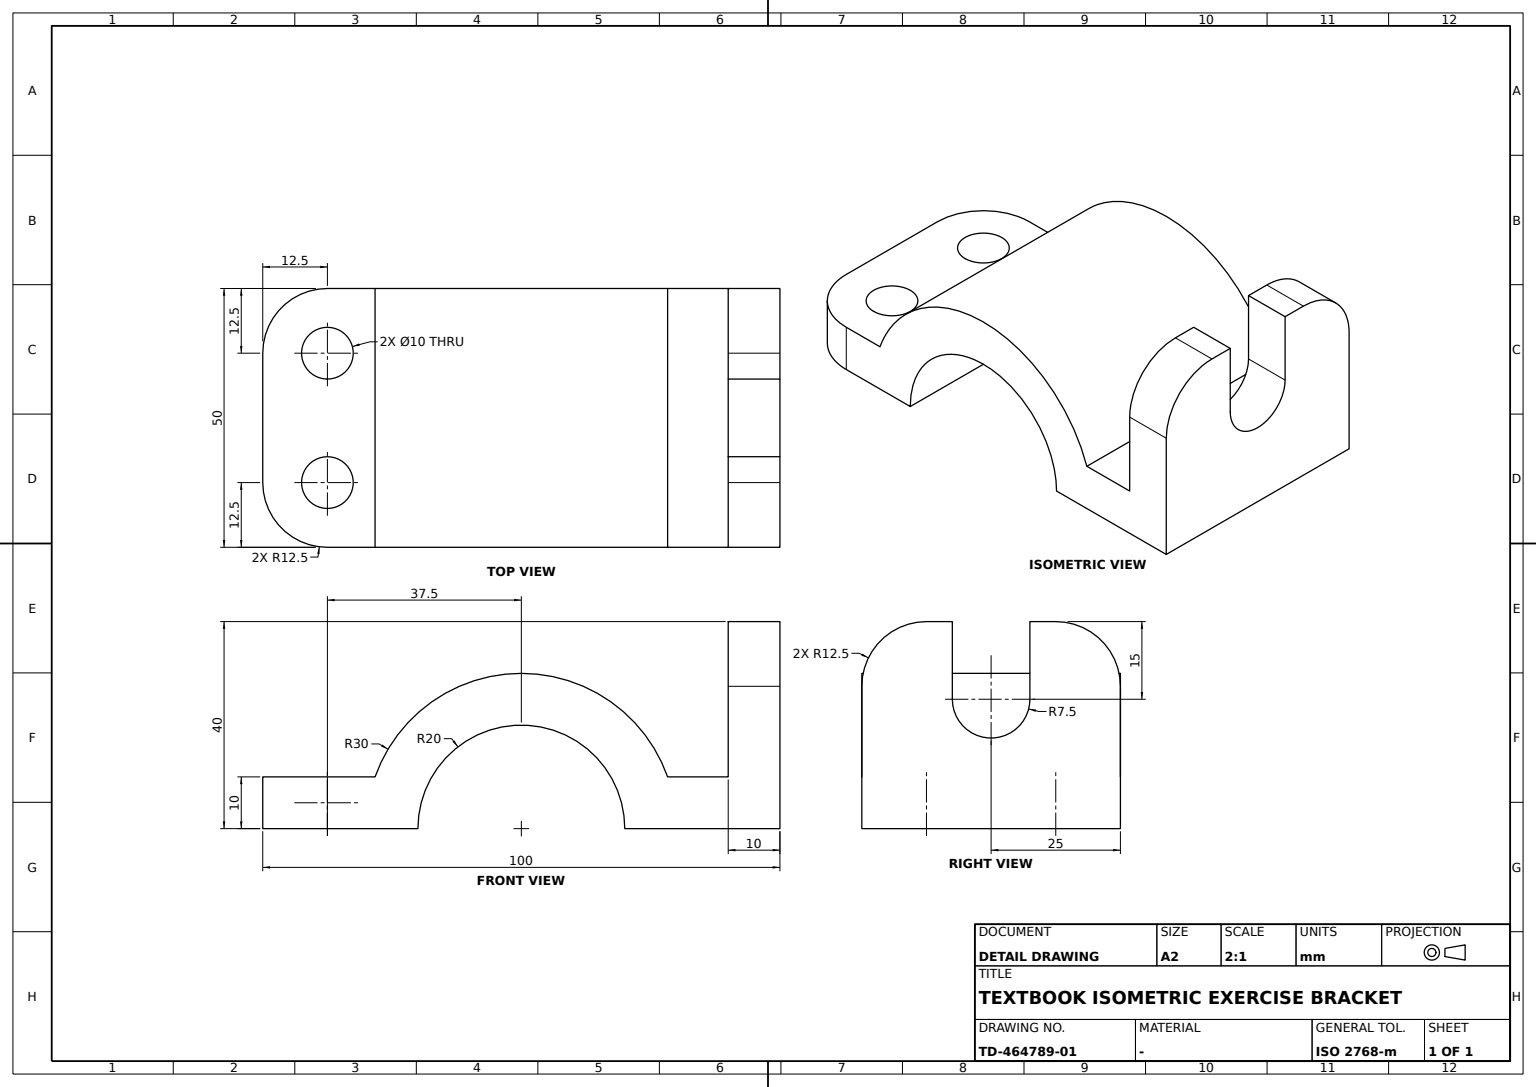
ISO-10303-21;
HEADER;
FILE_DESCRIPTION((''),'2;1');
FILE_NAME('','',(''),(''),'','','');
FILE_SCHEMA(('AUTOMOTIVE_DESIGN'));
ENDSEC;
DATA;
#1=APPLICATION_CONTEXT('');
#2=PRODUCT_CONTEXT('',#1,'mechanical');
#3=PRODUCT('','','',(#2));
#4=PRODUCT_DEFINITION_FORMATION('','',#3);
#5=PRODUCT_DEFINITION_CONTEXT('',#1,'design');
#6=PRODUCT_DEFINITION('','',#4,#5);
#7=PRODUCT_DEFINITION_SHAPE('','',#6);
#8=(LENGTH_UNIT()NAMED_UNIT(*)SI_UNIT(.MILLI.,.METRE.));
#9=(NAMED_UNIT(*)PLANE_ANGLE_UNIT()SI_UNIT($,.RADIAN.));
#10=(NAMED_UNIT(*)SI_UNIT($,.STERADIAN.)SOLID_ANGLE_UNIT());
#11=UNCERTAINTY_MEASURE_WITH_UNIT(LENGTH_MEASURE(1.E-05),#8,'distance_accuracy_value','');
#12=(GEOMETRIC_REPRESENTATION_CONTEXT(3)GLOBAL_UNCERTAINTY_ASSIGNED_CONTEXT((#11))GLOBAL_UNIT_ASSIGNED_CONTEXT((#8,#9,#10))REPRESENTATION_CONTEXT('',''));
#13=CARTESIAN_POINT('',(12.5,40.,40.));
#14=VERTEX_POINT('',#13);
#15=CARTESIAN_POINT('',(25.,40.,27.5));
#16=VERTEX_POINT('',#15);
#17=CARTESIAN_POINT('',(12.5,40.,27.5));
#18=DIRECTION('',(0.,1.,0.));
#19=DIRECTION('',(0.,0.,-1.));
#20=AXIS2_PLACEMENT_3D('',#17,#18,#19);
#21=CIRCLE('',#20,12.5);
#22=EDGE_CURVE('',#14,#16,#21,.T.);
#23=ORIENTED_EDGE('',*,*,#22,.F.);
#24=CARTESIAN_POINT('',(7.5,40.,40.));
#25=VERTEX_POINT('',#24);
#26=CARTESIAN_POINT('',(10.,40.,40.));
#27=DIRECTION('',(1.,0.,0.));
#28=VECTOR('',#27,1000.);
#29=LINE('',#26,#28);
#30=EDGE_CURVE('',#25,#14,#29,.T.);
#31=ORIENTED_EDGE('',*,*,#30,.F.);
#32=CARTESIAN_POINT('',(7.5,40.,25.));
#33=VERTEX_POINT('',#32);
#34=CARTESIAN_POINT('',(7.5,40.,32.5));
#35=VECTOR('',#19,1000.);
#36=LINE('',#34,#35);
#37=EDGE_CURVE('',#25,#33,#36,.T.);
#38=ORIENTED_EDGE('',*,*,#37,.T.);
#39=CARTESIAN_POINT('',(-7.5,40.,25.));
#40=VERTEX_POINT('',#39);
#41=CARTESIAN_POINT('',(0.,40.,25.));
#42=DIRECTION('',(0.,-1.,0.));
#43=AXIS2_PLACEMENT_3D('',#41,#42,#19);
#44=CIRCLE('',#43,7.5);
#45=EDGE_CURVE('',#40,#33,#44,.T.);
#46=ORIENTED_EDGE('',*,*,#45,.F.);
#47=CARTESIAN_POINT('',(-7.5,40.,40.));
#48=VERTEX_POINT('',#47);
#49=CARTESIAN_POINT('',(-7.5,40.,32.5));
#50=LINE('',#49,#35);
#51=EDGE_CURVE('',#48,#40,#50,.T.);
#52=ORIENTED_EDGE('',*,*,#51,.F.);
#53=CARTESIAN_POINT('',(-12.5,40.,40.));
#54=VERTEX_POINT('',#53);
#55=CARTESIAN_POINT('',(-10.,40.,40.));
#56=LINE('',#55,#28);
#57=EDGE_CURVE('',#54,#48,#56,.T.);
#58=ORIENTED_EDGE('',*,*,#57,.F.);
#59=CARTESIAN_POINT('',(-25.,40.,27.5));
#60=VERTEX_POINT('',#59);
#61=CARTESIAN_POINT('',(-12.5,40.,27.5));
#62=AXIS2_PLACEMENT_3D('',#61,#18,#19);
#63=CIRCLE('',#62,12.5);
#64=EDGE_CURVE('',#60,#54,#63,.T.);
#65=ORIENTED_EDGE('',*,*,#64,.F.);
#66=CARTESIAN_POINT('',(-25.,40.,10.));
#67=VERTEX_POINT('',#66);
#68=CARTESIAN_POINT('',(-25.,40.,18.75));
#69=LINE('',#68,#35);
#70=EDGE_CURVE('',#60,#67,#69,.T.);
#71=ORIENTED_EDGE('',*,*,#70,.T.);
#72=CARTESIAN_POINT('',(25.,40.,10.));
#73=VERTEX_POINT('',#72);
#74=CARTESIAN_POINT('',(0.,40.,10.));
#75=LINE('',#74,#28);
#76=EDGE_CURVE('',#67,#73,#75,.T.);
#77=ORIENTED_EDGE('',*,*,#76,.T.);
#78=CARTESIAN_POINT('',(25.,40.,18.75));
#79=LINE('',#78,#35);
#80=EDGE_CURVE('',#16,#73,#79,.T.);
#81=ORIENTED_EDGE('',*,*,#80,.F.);
#82=EDGE_LOOP('',(#23,#31,#38,#46,#52,#58,#65,#71,#77,#81));
#83=FACE_OUTER_BOUND('',#82,.T.);
#84=CARTESIAN_POINT('',(0.,40.,40.));
#85=AXIS2_PLACEMENT_3D('',#84,#42,#19);
#86=PLANE('',#85);
#87=ADVANCED_FACE('',(#83),#86,.T.);
#88=CARTESIAN_POINT('',(-25.,-37.5,0.));
#89=VERTEX_POINT('',#88);
#90=CARTESIAN_POINT('',(-12.5,-50.,0.));
#91=VERTEX_POINT('',#90);
#92=CARTESIAN_POINT('',(-12.5,-37.5,0.));
#93=DIRECTION('',(0.,0.,1.));
#94=AXIS2_PLACEMENT_3D('',#92,#93,#18);
#95=CIRCLE('',#94,12.5);
#96=EDGE_CURVE('',#89,#91,#95,.T.);
#97=ORIENTED_EDGE('',*,*,#96,.T.);
#98=CARTESIAN_POINT('',(-12.5,-50.,10.));
#99=VERTEX_POINT('',#98);
#100=CARTESIAN_POINT('',(-12.5,-50.,5.));
#101=LINE('',#100,#35);
#102=EDGE_CURVE('',#99,#91,#101,.T.);
#103=ORIENTED_EDGE('',*,*,#102,.F.);
#104=CARTESIAN_POINT('',(-25.,-37.5,10.));
#105=VERTEX_POINT('',#104);
#106=CARTESIAN_POINT('',(-12.5,-37.5,10.));
#107=AXIS2_PLACEMENT_3D('',#106,#19,#42);
#108=CIRCLE('',#107,12.5);
#109=EDGE_CURVE('',#99,#105,#108,.T.);
#110=ORIENTED_EDGE('',*,*,#109,.T.);
#111=CARTESIAN_POINT('',(-25.,-37.5,5.));
#112=LINE('',#111,#35);
#113=EDGE_CURVE('',#105,#89,#112,.T.);
#114=ORIENTED_EDGE('',*,*,#113,.T.);
#115=EDGE_LOOP('',(#97,#103,#110,#114));
#116=FACE_OUTER_BOUND('',#115,.T.);
#117=CARTESIAN_POINT('',(-12.5,-37.5,15.));
#118=DIRECTION('',(-1.,0.,0.));
#119=AXIS2_PLACEMENT_3D('',#117,#19,#118);
#120=CYLINDRICAL_SURFACE('',#119,12.5);
#121=ADVANCED_FACE('',(#116),#120,.T.);
#122=CARTESIAN_POINT('',(17.5,-37.5,0.));
#123=VERTEX_POINT('',#122);
#124=CARTESIAN_POINT('',(7.5,-37.5,0.));
#125=VERTEX_POINT('',#124);
#126=CARTESIAN_POINT('',(12.5,-37.5,0.));
#127=AXIS2_PLACEMENT_3D('',#126,#19,#18);
#128=CIRCLE('',#127,5.);
#129=EDGE_CURVE('',#123,#125,#128,.T.);
#130=ORIENTED_EDGE('',*,*,#129,.T.);
#131=CARTESIAN_POINT('',(7.5,-37.5,10.));
#132=VERTEX_POINT('',#131);
#133=CARTESIAN_POINT('',(7.5,-37.5,-2.5));
#134=LINE('',#133,#35);
#135=EDGE_CURVE('',#132,#125,#134,.T.);
#136=ORIENTED_EDGE('',*,*,#135,.F.);
#137=CARTESIAN_POINT('',(17.5,-37.5,10.));
#138=VERTEX_POINT('',#137);
#139=CARTESIAN_POINT('',(12.5,-37.5,10.));
#140=AXIS2_PLACEMENT_3D('',#139,#93,#27);
#141=CIRCLE('',#140,5.);
#142=EDGE_CURVE('',#132,#138,#141,.T.);
#143=ORIENTED_EDGE('',*,*,#142,.T.);
#144=CARTESIAN_POINT('',(17.5,-37.5,-2.5));
#145=LINE('',#144,#35);
#146=EDGE_CURVE('',#138,#123,#145,.T.);
#147=ORIENTED_EDGE('',*,*,#146,.T.);
#148=EDGE_LOOP('',(#130,#136,#143,#147));
#149=FACE_OUTER_BOUND('',#148,.T.);
#150=CARTESIAN_POINT('',(12.5,-37.5,-2.5));
#151=AXIS2_PLACEMENT_3D('',#150,#19,#27);
#152=CYLINDRICAL_SURFACE('',#151,5.);
#153=ADVANCED_FACE('',(#149),#152,.F.);
#154=CARTESIAN_POINT('',(12.5,50.,40.));
#155=VERTEX_POINT('',#154);
#156=CARTESIAN_POINT('',(12.5,45.,40.));
#157=VECTOR('',#42,1000.);
#158=LINE('',#156,#157);
#159=EDGE_CURVE('',#155,#14,#158,.T.);
#160=ORIENTED_EDGE('',*,*,#159,.T.);
#161=ORIENTED_EDGE('',*,*,#22,.T.);
#162=CARTESIAN_POINT('',(25.,50.,27.5));
#163=VERTEX_POINT('',#162);
#164=CARTESIAN_POINT('',(25.,45.,27.5));
#165=LINE('',#164,#157);
#166=EDGE_CURVE('',#163,#16,#165,.T.);
#167=ORIENTED_EDGE('',*,*,#166,.F.);
#168=CARTESIAN_POINT('',(12.5,50.,27.5));
#169=AXIS2_PLACEMENT_3D('',#168,#42,#93);
#170=CIRCLE('',#169,12.5);
#171=EDGE_CURVE('',#163,#155,#170,.T.);
#172=ORIENTED_EDGE('',*,*,#171,.T.);
#173=EDGE_LOOP('',(#160,#161,#167,#172));
#174=FACE_OUTER_BOUND('',#173,.T.);
#175=CARTESIAN_POINT('',(12.5,0.,27.5));
#176=AXIS2_PLACEMENT_3D('',#175,#18,#93);
#177=CYLINDRICAL_SURFACE('',#176,12.5);
#178=ADVANCED_FACE('',(#174),#177,.T.);
#179=CARTESIAN_POINT('',(12.5,-50.,0.));
#180=VERTEX_POINT('',#179);
#181=CARTESIAN_POINT('',(25.,-37.5,0.));
#182=VERTEX_POINT('',#181);
#183=AXIS2_PLACEMENT_3D('',#126,#93,#18);
#184=CIRCLE('',#183,12.5);
#185=EDGE_CURVE('',#180,#182,#184,.T.);
#186=ORIENTED_EDGE('',*,*,#185,.T.);
#187=CARTESIAN_POINT('',(25.,-37.5,10.));
#188=VERTEX_POINT('',#187);
#189=CARTESIAN_POINT('',(25.,-37.5,5.));
#190=LINE('',#189,#35);
#191=EDGE_CURVE('',#188,#182,#190,.T.);
#192=ORIENTED_EDGE('',*,*,#191,.F.);
#193=CARTESIAN_POINT('',(12.5,-50.,10.));
#194=VERTEX_POINT('',#193);
#195=AXIS2_PLACEMENT_3D('',#139,#19,#42);
#196=CIRCLE('',#195,12.5);
#197=EDGE_CURVE('',#188,#194,#196,.T.);
#198=ORIENTED_EDGE('',*,*,#197,.T.);
#199=CARTESIAN_POINT('',(12.5,-50.,5.));
#200=LINE('',#199,#35);
#201=EDGE_CURVE('',#194,#180,#200,.T.);
#202=ORIENTED_EDGE('',*,*,#201,.T.);
#203=EDGE_LOOP('',(#186,#192,#198,#202));
#204=FACE_OUTER_BOUND('',#203,.T.);
#205=CARTESIAN_POINT('',(12.5,-37.5,15.));
#206=AXIS2_PLACEMENT_3D('',#205,#19,#42);
#207=CYLINDRICAL_SURFACE('',#206,12.5);
#208=ADVANCED_FACE('',(#204),#207,.T.);
#209=CARTESIAN_POINT('',(0.,-50.,0.));
#210=LINE('',#209,#28);
#211=EDGE_CURVE('',#91,#180,#210,.T.);
#212=ORIENTED_EDGE('',*,*,#211,.T.);
#213=ORIENTED_EDGE('',*,*,#201,.F.);
#214=CARTESIAN_POINT('',(0.,-50.,10.));
#215=LINE('',#214,#28);
#216=EDGE_CURVE('',#99,#194,#215,.T.);
#217=ORIENTED_EDGE('',*,*,#216,.F.);
#218=ORIENTED_EDGE('',*,*,#102,.T.);
#219=EDGE_LOOP('',(#212,#213,#217,#218));
#220=FACE_OUTER_BOUND('',#219,.T.);
#221=AXIS2_PLACEMENT_3D('',#209,#18,#93);
#222=PLANE('',#221);
#223=ADVANCED_FACE('',(#220),#222,.F.);
#224=CARTESIAN_POINT('',(7.5,50.,40.));
#225=VERTEX_POINT('',#224);
#226=CARTESIAN_POINT('',(7.5,50.,25.));
#227=VERTEX_POINT('',#226);
#228=CARTESIAN_POINT('',(7.5,50.,32.5));
#229=LINE('',#228,#35);
#230=EDGE_CURVE('',#225,#227,#229,.T.);
#231=ORIENTED_EDGE('',*,*,#230,.F.);
#232=CARTESIAN_POINT('',(10.,50.,40.));
#233=LINE('',#232,#28);
#234=EDGE_CURVE('',#225,#155,#233,.T.);
#235=ORIENTED_EDGE('',*,*,#234,.T.);
#236=ORIENTED_EDGE('',*,*,#171,.F.);
#237=CARTESIAN_POINT('',(25.,50.,0.));
#238=VERTEX_POINT('',#237);
#239=CARTESIAN_POINT('',(25.,50.,13.75));
#240=VECTOR('',#93,1000.);
#241=LINE('',#239,#240);
#242=EDGE_CURVE('',#238,#163,#241,.T.);
#243=ORIENTED_EDGE('',*,*,#242,.F.);
#244=CARTESIAN_POINT('',(-25.,50.,0.));
#245=VERTEX_POINT('',#244);
#246=CARTESIAN_POINT('',(0.,50.,0.));
#247=LINE('',#246,#28);
#248=EDGE_CURVE('',#245,#238,#247,.T.);
#249=ORIENTED_EDGE('',*,*,#248,.F.);
#250=CARTESIAN_POINT('',(-25.,50.,27.5));
#251=VERTEX_POINT('',#250);
#252=CARTESIAN_POINT('',(-25.,50.,13.75));
#253=LINE('',#252,#240);
#254=EDGE_CURVE('',#245,#251,#253,.T.);
#255=ORIENTED_EDGE('',*,*,#254,.T.);
#256=CARTESIAN_POINT('',(-12.5,50.,40.));
#257=VERTEX_POINT('',#256);
#258=CARTESIAN_POINT('',(-12.5,50.,27.5));
#259=AXIS2_PLACEMENT_3D('',#258,#42,#93);
#260=CIRCLE('',#259,12.5);
#261=EDGE_CURVE('',#257,#251,#260,.T.);
#262=ORIENTED_EDGE('',*,*,#261,.F.);
#263=CARTESIAN_POINT('',(-7.5,50.,40.));
#264=VERTEX_POINT('',#263);
#265=CARTESIAN_POINT('',(-10.,50.,40.));
#266=LINE('',#265,#28);
#267=EDGE_CURVE('',#257,#264,#266,.T.);
#268=ORIENTED_EDGE('',*,*,#267,.T.);
#269=CARTESIAN_POINT('',(-7.5,50.,25.));
#270=VERTEX_POINT('',#269);
#271=CARTESIAN_POINT('',(-7.5,50.,32.5));
#272=LINE('',#271,#240);
#273=EDGE_CURVE('',#270,#264,#272,.T.);
#274=ORIENTED_EDGE('',*,*,#273,.F.);
#275=CARTESIAN_POINT('',(0.,50.,25.));
#276=AXIS2_PLACEMENT_3D('',#275,#18,#118);
#277=CIRCLE('',#276,7.5);
#278=EDGE_CURVE('',#227,#270,#277,.T.);
#279=ORIENTED_EDGE('',*,*,#278,.F.);
#280=EDGE_LOOP('',(#231,#235,#236,#243,#249,#255,#262,#268,#274,#279));
#281=FACE_OUTER_BOUND('',#280,.T.);
#282=AXIS2_PLACEMENT_3D('',#246,#18,#93);
#283=PLANE('',#282);
#284=ADVANCED_FACE('',(#281),#283,.T.);
#285=CARTESIAN_POINT('',(25.,-20.,0.));
#286=VERTEX_POINT('',#285);
#287=CARTESIAN_POINT('',(25.,-28.75,0.));
#288=VECTOR('',#18,1000.);
#289=LINE('',#287,#288);
#290=EDGE_CURVE('',#182,#286,#289,.T.);
#291=ORIENTED_EDGE('',*,*,#290,.T.);
#292=CARTESIAN_POINT('',(25.,20.,0.));
#293=VERTEX_POINT('',#292);
#294=CARTESIAN_POINT('',(25.,0.,0.));
#295=AXIS2_PLACEMENT_3D('',#294,#118,#18);
#296=CIRCLE('',#295,20.);
#297=EDGE_CURVE('',#286,#293,#296,.T.);
#298=ORIENTED_EDGE('',*,*,#297,.T.);
#299=CARTESIAN_POINT('',(25.,35.,0.));
#300=LINE('',#299,#288);
#301=EDGE_CURVE('',#293,#238,#300,.T.);
#302=ORIENTED_EDGE('',*,*,#301,.T.);
#303=ORIENTED_EDGE('',*,*,#242,.T.);
#304=ORIENTED_EDGE('',*,*,#166,.T.);
#305=ORIENTED_EDGE('',*,*,#80,.T.);
#306=CARTESIAN_POINT('',(25.,28.284271,10.));
#307=VERTEX_POINT('',#306);
#308=CARTESIAN_POINT('',(25.,34.142136,10.));
#309=LINE('',#308,#157);
#310=EDGE_CURVE('',#73,#307,#309,.T.);
#311=ORIENTED_EDGE('',*,*,#310,.T.);
#312=CARTESIAN_POINT('',(25.,-28.284271,10.));
#313=VERTEX_POINT('',#312);
#314=AXIS2_PLACEMENT_3D('',#294,#27,#18);
#315=CIRCLE('',#314,30.);
#316=EDGE_CURVE('',#307,#313,#315,.T.);
#317=ORIENTED_EDGE('',*,*,#316,.T.);
#318=CARTESIAN_POINT('',(25.,-32.892136,10.));
#319=LINE('',#318,#157);
#320=EDGE_CURVE('',#313,#188,#319,.T.);
#321=ORIENTED_EDGE('',*,*,#320,.T.);
#322=ORIENTED_EDGE('',*,*,#191,.T.);
#323=EDGE_LOOP('',(#291,#298,#302,#303,#304,#305,#311,#317,#321,#322));
#324=FACE_OUTER_BOUND('',#323,.T.);
#325=PLANE('',#314);
#326=ADVANCED_FACE('',(#324),#325,.T.);
#327=ORIENTED_EDGE('',*,*,#278,.T.);
#328=CARTESIAN_POINT('',(-7.5,-0.66,25.));
#329=LINE('',#328,#157);
#330=EDGE_CURVE('',#270,#40,#329,.T.);
#331=ORIENTED_EDGE('',*,*,#330,.T.);
#332=ORIENTED_EDGE('',*,*,#45,.T.);
#333=CARTESIAN_POINT('',(7.5,45.,25.));
#334=LINE('',#333,#157);
#335=EDGE_CURVE('',#227,#33,#334,.T.);
#336=ORIENTED_EDGE('',*,*,#335,.F.);
#337=EDGE_LOOP('',(#327,#331,#332,#336));
#338=FACE_OUTER_BOUND('',#337,.T.);
#339=CARTESIAN_POINT('',(0.,-0.66,25.));
#340=AXIS2_PLACEMENT_3D('',#339,#42,#118);
#341=CYLINDRICAL_SURFACE('',#340,7.5);
#342=ADVANCED_FACE('',(#338),#341,.F.);
#343=EDGE_CURVE('',#138,#132,#141,.T.);
#344=ORIENTED_EDGE('',*,*,#343,.T.);
#345=ORIENTED_EDGE('',*,*,#135,.T.);
#346=EDGE_CURVE('',#125,#123,#128,.T.);
#347=ORIENTED_EDGE('',*,*,#346,.T.);
#348=ORIENTED_EDGE('',*,*,#146,.F.);
#349=EDGE_LOOP('',(#344,#345,#347,#348));
#350=FACE_OUTER_BOUND('',#349,.T.);
#351=ADVANCED_FACE('',(#350),#152,.F.);
#352=CARTESIAN_POINT('',(-12.5,45.,40.));
#353=LINE('',#352,#157);
#354=EDGE_CURVE('',#257,#54,#353,.T.);
#355=ORIENTED_EDGE('',*,*,#354,.T.);
#356=ORIENTED_EDGE('',*,*,#57,.T.);
#357=CARTESIAN_POINT('',(-7.5,45.,40.));
#358=LINE('',#357,#157);
#359=EDGE_CURVE('',#264,#48,#358,.T.);
#360=ORIENTED_EDGE('',*,*,#359,.F.);
#361=ORIENTED_EDGE('',*,*,#267,.F.);
#362=EDGE_LOOP('',(#355,#356,#360,#361));
#363=FACE_OUTER_BOUND('',#362,.T.);
#364=CARTESIAN_POINT('',(0.,50.,40.));
#365=AXIS2_PLACEMENT_3D('',#364,#93,#42);
#366=PLANE('',#365);
#367=ADVANCED_FACE('',(#363),#366,.T.);
#368=ORIENTED_EDGE('',*,*,#310,.F.);
#369=ORIENTED_EDGE('',*,*,#76,.F.);
#370=CARTESIAN_POINT('',(-25.,28.284271,10.));
#371=VERTEX_POINT('',#370);
#372=CARTESIAN_POINT('',(-25.,34.142136,10.));
#373=LINE('',#372,#157);
#374=EDGE_CURVE('',#67,#371,#373,.T.);
#375=ORIENTED_EDGE('',*,*,#374,.T.);
#376=CARTESIAN_POINT('',(0.,28.284271,10.));
#377=LINE('',#376,#28);
#378=EDGE_CURVE('',#371,#307,#377,.T.);
#379=ORIENTED_EDGE('',*,*,#378,.T.);
#380=EDGE_LOOP('',(#368,#369,#375,#379));
#381=FACE_OUTER_BOUND('',#380,.T.);
#382=AXIS2_PLACEMENT_3D('',#74,#93,#42);
#383=PLANE('',#382);
#384=ADVANCED_FACE('',(#381),#383,.T.);
#385=ORIENTED_EDGE('',*,*,#37,.F.);
#386=CARTESIAN_POINT('',(7.5,45.,40.));
#387=LINE('',#386,#157);
#388=EDGE_CURVE('',#225,#25,#387,.T.);
#389=ORIENTED_EDGE('',*,*,#388,.F.);
#390=ORIENTED_EDGE('',*,*,#230,.T.);
#391=ORIENTED_EDGE('',*,*,#335,.T.);
#392=EDGE_LOOP('',(#385,#389,#390,#391));
#393=FACE_OUTER_BOUND('',#392,.T.);
#394=AXIS2_PLACEMENT_3D('',#224,#118,#19);
#395=PLANE('',#394);
#396=ADVANCED_FACE('',(#393),#395,.T.);
#397=ORIENTED_EDGE('',*,*,#330,.F.);
#398=ORIENTED_EDGE('',*,*,#273,.T.);
#399=ORIENTED_EDGE('',*,*,#359,.T.);
#400=ORIENTED_EDGE('',*,*,#51,.T.);
#401=EDGE_LOOP('',(#397,#398,#399,#400));
#402=FACE_OUTER_BOUND('',#401,.T.);
#403=AXIS2_PLACEMENT_3D('',#263,#118,#19);
#404=PLANE('',#403);
#405=ADVANCED_FACE('',(#402),#404,.F.);
#406=CARTESIAN_POINT('',(-25.,20.,0.));
#407=VERTEX_POINT('',#406);
#408=CARTESIAN_POINT('',(-25.,35.,0.));
#409=LINE('',#408,#288);
#410=EDGE_CURVE('',#407,#245,#409,.T.);
#411=ORIENTED_EDGE('',*,*,#410,.F.);
#412=CARTESIAN_POINT('',(-25.,-20.,0.));
#413=VERTEX_POINT('',#412);
#414=CARTESIAN_POINT('',(-25.,0.,0.));
#415=AXIS2_PLACEMENT_3D('',#414,#118,#18);
#416=CIRCLE('',#415,20.);
#417=EDGE_CURVE('',#413,#407,#416,.T.);
#418=ORIENTED_EDGE('',*,*,#417,.F.);
#419=CARTESIAN_POINT('',(-25.,-28.75,0.));
#420=LINE('',#419,#288);
#421=EDGE_CURVE('',#89,#413,#420,.T.);
#422=ORIENTED_EDGE('',*,*,#421,.F.);
#423=ORIENTED_EDGE('',*,*,#113,.F.);
#424=CARTESIAN_POINT('',(-25.,-28.284271,10.));
#425=VERTEX_POINT('',#424);
#426=CARTESIAN_POINT('',(-25.,-32.892136,10.));
#427=LINE('',#426,#157);
#428=EDGE_CURVE('',#425,#105,#427,.T.);
#429=ORIENTED_EDGE('',*,*,#428,.F.);
#430=AXIS2_PLACEMENT_3D('',#414,#27,#18);
#431=CIRCLE('',#430,30.);
#432=EDGE_CURVE('',#371,#425,#431,.T.);
#433=ORIENTED_EDGE('',*,*,#432,.F.);
#434=ORIENTED_EDGE('',*,*,#374,.F.);
#435=ORIENTED_EDGE('',*,*,#70,.F.);
#436=CARTESIAN_POINT('',(-25.,45.,27.5));
#437=LINE('',#436,#157);
#438=EDGE_CURVE('',#251,#60,#437,.T.);
#439=ORIENTED_EDGE('',*,*,#438,.F.);
#440=ORIENTED_EDGE('',*,*,#254,.F.);
#441=EDGE_LOOP('',(#411,#418,#422,#423,#429,#433,#434,#435,#439,#440));
#442=FACE_OUTER_BOUND('',#441,.T.);
#443=PLANE('',#430);
#444=ADVANCED_FACE('',(#442),#443,.F.);
#445=ORIENTED_EDGE('',*,*,#261,.T.);
#446=ORIENTED_EDGE('',*,*,#438,.T.);
#447=ORIENTED_EDGE('',*,*,#64,.T.);
#448=ORIENTED_EDGE('',*,*,#354,.F.);
#449=EDGE_LOOP('',(#445,#446,#447,#448));
#450=FACE_OUTER_BOUND('',#449,.T.);
#451=CARTESIAN_POINT('',(-12.5,0.,27.5));
#452=AXIS2_PLACEMENT_3D('',#451,#18,#118);
#453=CYLINDRICAL_SURFACE('',#452,12.5);
#454=ADVANCED_FACE('',(#450),#453,.T.);
#455=ORIENTED_EDGE('',*,*,#159,.F.);
#456=ORIENTED_EDGE('',*,*,#234,.F.);
#457=ORIENTED_EDGE('',*,*,#388,.T.);
#458=ORIENTED_EDGE('',*,*,#30,.T.);
#459=EDGE_LOOP('',(#455,#456,#457,#458));
#460=FACE_OUTER_BOUND('',#459,.T.);
#461=ADVANCED_FACE('',(#460),#366,.T.);
#462=CARTESIAN_POINT('',(-17.5,-37.5,10.));
#463=VERTEX_POINT('',#462);
#464=CARTESIAN_POINT('',(-17.5,-37.5,0.));
#465=VERTEX_POINT('',#464);
#466=CARTESIAN_POINT('',(-17.5,-37.5,-2.5));
#467=LINE('',#466,#35);
#468=EDGE_CURVE('',#463,#465,#467,.T.);
#469=ORIENTED_EDGE('',*,*,#468,.T.);
#470=CARTESIAN_POINT('',(-7.5,-37.5,0.));
#471=VERTEX_POINT('',#470);
#472=AXIS2_PLACEMENT_3D('',#92,#19,#18);
#473=CIRCLE('',#472,5.);
#474=EDGE_CURVE('',#465,#471,#473,.T.);
#475=ORIENTED_EDGE('',*,*,#474,.T.);
#476=CARTESIAN_POINT('',(-7.5,-37.5,10.));
#477=VERTEX_POINT('',#476);
#478=CARTESIAN_POINT('',(-7.5,-37.5,-2.5));
#479=LINE('',#478,#35);
#480=EDGE_CURVE('',#477,#471,#479,.T.);
#481=ORIENTED_EDGE('',*,*,#480,.F.);
#482=AXIS2_PLACEMENT_3D('',#106,#93,#27);
#483=CIRCLE('',#482,5.);
#484=EDGE_CURVE('',#477,#463,#483,.T.);
#485=ORIENTED_EDGE('',*,*,#484,.T.);
#486=EDGE_LOOP('',(#469,#475,#481,#485));
#487=FACE_OUTER_BOUND('',#486,.T.);
#488=CARTESIAN_POINT('',(-12.5,-37.5,-2.5));
#489=AXIS2_PLACEMENT_3D('',#488,#19,#27);
#490=CYLINDRICAL_SURFACE('',#489,5.);
#491=ADVANCED_FACE('',(#487),#490,.F.);
#492=EDGE_CURVE('',#463,#477,#483,.T.);
#493=ORIENTED_EDGE('',*,*,#492,.T.);
#494=ORIENTED_EDGE('',*,*,#480,.T.);
#495=EDGE_CURVE('',#471,#465,#473,.T.);
#496=ORIENTED_EDGE('',*,*,#495,.T.);
#497=ORIENTED_EDGE('',*,*,#468,.F.);
#498=EDGE_LOOP('',(#493,#494,#496,#497));
#499=FACE_OUTER_BOUND('',#498,.T.);
#500=ADVANCED_FACE('',(#499),#490,.F.);
#501=ORIENTED_EDGE('',*,*,#297,.F.);
#502=CARTESIAN_POINT('',(0.,-20.,0.));
#503=LINE('',#502,#28);
#504=EDGE_CURVE('',#413,#286,#503,.T.);
#505=ORIENTED_EDGE('',*,*,#504,.F.);
#506=ORIENTED_EDGE('',*,*,#417,.T.);
#507=CARTESIAN_POINT('',(0.,20.,0.));
#508=LINE('',#507,#28);
#509=EDGE_CURVE('',#407,#293,#508,.T.);
#510=ORIENTED_EDGE('',*,*,#509,.T.);
#511=EDGE_LOOP('',(#501,#505,#506,#510));
#512=FACE_OUTER_BOUND('',#511,.T.);
#513=CARTESIAN_POINT('',(0.,0.,0.));
#514=AXIS2_PLACEMENT_3D('',#513,#118,#18);
#515=CYLINDRICAL_SURFACE('',#514,20.);
#516=ADVANCED_FACE('',(#512),#515,.F.);
#517=ORIENTED_EDGE('',*,*,#495,.F.);
#518=ORIENTED_EDGE('',*,*,#474,.F.);
#519=EDGE_LOOP('',(#517,#518));
#520=FACE_BOUND('',#519,.T.);
#521=ORIENTED_EDGE('',*,*,#346,.F.);
#522=ORIENTED_EDGE('',*,*,#129,.F.);
#523=EDGE_LOOP('',(#521,#522));
#524=FACE_BOUND('',#523,.T.);
#525=ORIENTED_EDGE('',*,*,#211,.F.);
#526=ORIENTED_EDGE('',*,*,#96,.F.);
#527=ORIENTED_EDGE('',*,*,#421,.T.);
#528=ORIENTED_EDGE('',*,*,#504,.T.);
#529=ORIENTED_EDGE('',*,*,#290,.F.);
#530=ORIENTED_EDGE('',*,*,#185,.F.);
#531=EDGE_LOOP('',(#525,#526,#527,#528,#529,#530));
#532=FACE_OUTER_BOUND('',#531,.T.);
#533=AXIS2_PLACEMENT_3D('',#507,#19,#18);
#534=PLANE('',#533);
#535=ADVANCED_FACE('',(#520,#524,#532),#534,.T.);
#536=ORIENTED_EDGE('',*,*,#484,.F.);
#537=ORIENTED_EDGE('',*,*,#492,.F.);
#538=EDGE_LOOP('',(#536,#537));
#539=FACE_BOUND('',#538,.T.);
#540=ORIENTED_EDGE('',*,*,#197,.F.);
#541=ORIENTED_EDGE('',*,*,#320,.F.);
#542=CARTESIAN_POINT('',(0.,-28.284271,10.));
#543=LINE('',#542,#28);
#544=EDGE_CURVE('',#425,#313,#543,.T.);
#545=ORIENTED_EDGE('',*,*,#544,.F.);
#546=ORIENTED_EDGE('',*,*,#428,.T.);
#547=ORIENTED_EDGE('',*,*,#109,.F.);
#548=ORIENTED_EDGE('',*,*,#216,.T.);
#549=EDGE_LOOP('',(#540,#541,#545,#546,#547,#548));
#550=FACE_OUTER_BOUND('',#549,.T.);
#551=ORIENTED_EDGE('',*,*,#142,.F.);
#552=ORIENTED_EDGE('',*,*,#343,.F.);
#553=EDGE_LOOP('',(#551,#552));
#554=FACE_BOUND('',#553,.T.);
#555=ADVANCED_FACE('',(#539,#550,#554),#383,.T.);
#556=ORIENTED_EDGE('',*,*,#410,.T.);
#557=ORIENTED_EDGE('',*,*,#248,.T.);
#558=ORIENTED_EDGE('',*,*,#301,.F.);
#559=ORIENTED_EDGE('',*,*,#509,.F.);
#560=EDGE_LOOP('',(#556,#557,#558,#559));
#561=FACE_OUTER_BOUND('',#560,.T.);
#562=ADVANCED_FACE('',(#561),#534,.T.);
#563=ORIENTED_EDGE('',*,*,#316,.F.);
#564=ORIENTED_EDGE('',*,*,#378,.F.);
#565=ORIENTED_EDGE('',*,*,#432,.T.);
#566=ORIENTED_EDGE('',*,*,#544,.T.);
#567=EDGE_LOOP('',(#563,#564,#565,#566));
#568=FACE_OUTER_BOUND('',#567,.T.);
#569=CYLINDRICAL_SURFACE('',#514,30.);
#570=ADVANCED_FACE('',(#568),#569,.T.);
#571=CLOSED_SHELL('',(#87,#121,#153,#178,#208,#223,#284,#326,#342,#351,#367,#384,#396,#405,#444,#454,#461,#491,#500,#516,#535,#555,#562,#570));
#572=MANIFOLD_SOLID_BREP('',#571);
#573=ADVANCED_BREP_SHAPE_REPRESENTATION('',(#572),#12);
#574=SHAPE_DEFINITION_REPRESENTATION(#7,#573);
ENDSEC;
END-ISO-10303-21;
